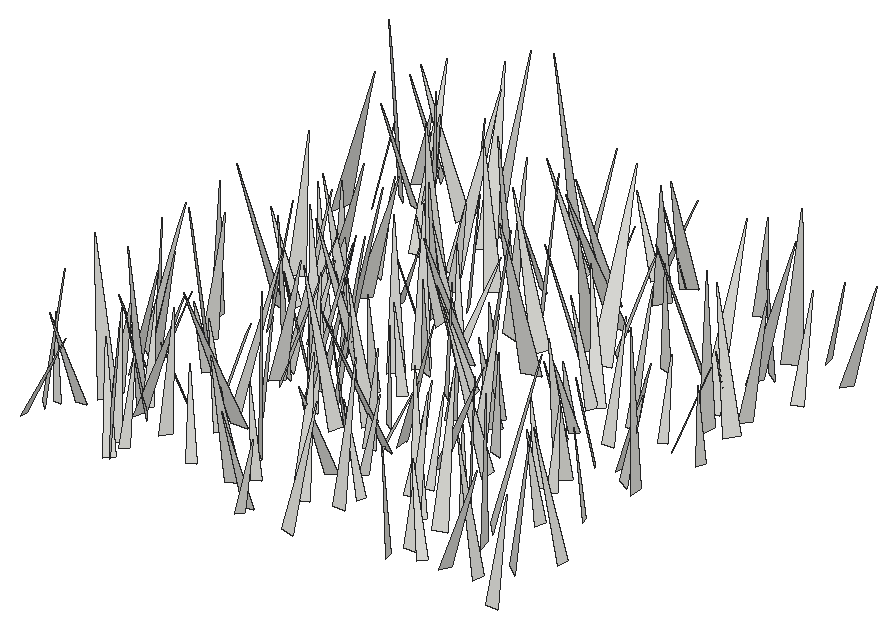
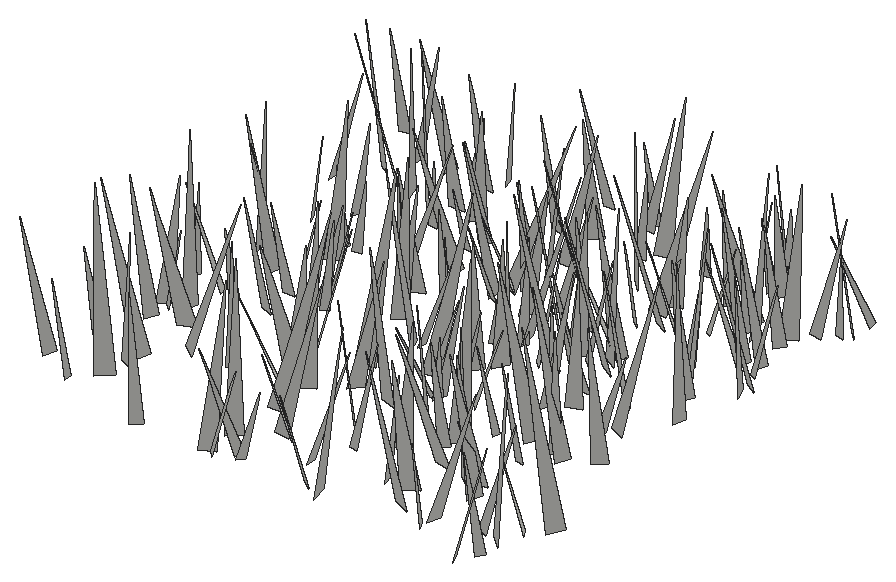
# SketchUp Ruby script. Lengths in inches.
U = 1.inch
M = Sketchup.active_model
def pt(a) = Geom::Point3d.new(a.map { |v| v * U })
def face(e, loops, mat)
  f = e.add_face(loops[0].map { |a| pt(a) })
  loops[1..].each { |l| e.add_face(l.map { |a| pt(a) }).erase! }
  f.material = f.back_material = mat if mat
  f
end
# faces: each face lists its corners as indices into pts; further lists are holes
def faces(e, pts, list, mat = nil) = list.each { |f| face(e, (f[0].is_a?(Array) ? f : [f]).map { |l| l.map { |i| pts[i] } }, mat) }
# xy, xz, yz: faces in a plane at the given z, y or x. An outline is a flat list of corners, or four numbers for a rectangle; further outlines are holes
def ring(l) = l.size == 4 ? [[l[0], l[1]], [l[2], l[1]], [l[2], l[3]], [l[0], l[3]]] : l.each_slice(2).to_a
def flat(e, list, mat, &to3) = list.each { |f| face(e, (f[0].is_a?(Array) ? f : [f]).map { |l| ring(l).map { |u, v| to3.(u, v) } }, mat) }
def xy(e, z, list, mat = nil) = flat(e, list, mat) { |x, y| [x, y, z] }
def xz(e, y, list, mat = nil) = flat(e, list, mat) { |x, z| [x, y, z] }
def yz(e, x, list, mat = nil) = flat(e, list, mat) { |y, z| [x, y, z] }
def lines(e, pts, list) = list.each { |a, b| e.add_line(pt(pts[a]), pt(pts[b])) }
# prism: a flat outline (further loops are holes) pulled along v
def prism(e, loops, v, mat = nil)
  f = face(e, loops, mat); d = Geom::Vector3d.new(v.map { |x| x * U })
  f.pushpull(f.normal.samedirection?(d) ? d.length : -d.length)
end
def box(e, o, s, mat = nil) = prism(e, [[o, [o[0] + s[0], o[1], o[2]], [o[0] + s[0], o[1] + s[1], o[2]], [o[0], o[1] + s[1], o[2]]]], [0, 0, s[2]], mat)
def at(x, y, z, deg = 0) = Geom::Transformation.translation(pt([x, y, z])) * Geom::Transformation.rotation(ORIGIN, Z_AXIS, deg.degrees)
def axes(o, x, y, z) = Geom::Transformation.new([*x, 0, *y, 0, *z, 0, *pt(o).to_a, 1])
def part(name) = M.definitions.add(name)
# library, detail: a bought-in or finely detailed component or shape, given as its bounding box
def library(name, o, s) = part(name).tap { |d| box(d.entities, o, s) }
def detail(e, o, s) = box(e.add_group.entities, o, s)
def put(e, d, t, mat = nil) = e.add_instance(d, t).tap { |i| i.material = mat if mat }
def group(e, t, mat = nil) = e.add_group.tap { |g| g.transformation = t; g.material = mat if mat }.entities
root = M.entities
c1 = part("fur_instance\#9")
p = [[0.8125,0,1.79],[0.67,-0.02,1.48],[0,-0.11,0],[0,0.11,0]]
faces(c1.entities,p,[[0,1,2,3]])
put(root,c1,axes([501.8,309.96,-21.66],[0.50374,3.60666,1.32904],[3.78488,-0.69911,0.46265],[-0.67011,-1.23747,3.61216]))
put(root,c1,axes([502.37,352.37,-21.66],[-4.94486,-5.49387,2.91837],[-6.02867,5.15162,-0.51692],[1.53451,2.53562,7.37341]))
put(root,c1,axes([501.12,309.07,-21.66],[4.60486,4.04407,1.88978],[4.30358,-4.74303,-0.33665],[-1.18533,-1.50984,6.1193]))
put(root,c1,axes([501.48,349.91,-21.66],[2.95559,2.2846,0.71516],[2.24296,-3.03986,0.44126],[-0.83663,-0.07885,3.70947]))
put(root,c1,axes([502.125,321.92,-21.66],[-4.83531,-1.63891,2.39644],[-2.01972,5.24312,-0.48946],[2.08559,1.27782,5.08199]))
put(root,c1,axes([503.12,356.64,-21.66],[-4.38014,-2.49103,0.91186],[-2.44951,4.47381,0.4553],[1.01814,0.04674,5.01832]))
put(root,c1,axes([499.65,348.23,-21.66],[8.0282,-2.33719,0.44231],[-2.30718,-8.02996,-0.55383],[-0.57877,-0.40914,8.34313]))
put(root,c1,axes([500.875,306.83,-21.66],[4.1398,0.29454,0.02134],[0.28882,-4.10074,0.57065],[-0.06159,0.56772,4.11084]))
put(root,c1,axes([503.16,319.11,-21.66],[-1.78915,-3.44674,0.35763],[-3.41457,1.82215,0.479],[0.59044,0.09337,3.85378]))
put(root,c1,axes([503.31,311.05,-21.66],[-0.2394,-4.99537,0.47277],[-5.01072,0.21306,-0.28607],[-0.26442,0.48521,4.99291]))
put(root,c1,axes([501.91,354.89,-21.66],[3.6262,-2.26105,0.60128],[-2.31235,-3.63241,0.28605],[-0.35624,0.56255,4.26378]))
put(root,c1,axes([501.99,320.76,-21.66],[3.861,5.57007,1.34937],[5.71182,-3.87341,-0.35436],[-0.47072,-1.31331,6.76812]))
put(root,c1,axes([504.14,351.86,-21.66],[-1.82389,-4.57282,0.8897],[-4.65371,1.74485,-0.5721],[-0.21262,1.03617,4.88978]))
put(root,c1,axes([503.1,328.43,-21.66],[6.40054,-0.55178,2.21578],[-0.37829,-6.75939,-0.5905],[-2.25189,-0.43282,6.39709]))
put(root,c1,axes([503.78,337.5625,-21.66],[3.27303,-4.65782,3.06275],[-5.40234,-3.52629,0.41046],[-1.37496,2.76738,5.67799]))
put(root,c1,axes([504.5625,312.82,-21.66],[-4.39266,5.33205,2.64396],[5.82364,4.52851,0.54275],[1.2274,-2.40386,6.88706]))
put(root,c1,axes([505.83,332.8,-21.66],[-2.53564,-6.45433,1.27855],[-6.57975,2.48748,-0.49186],[0.00081,1.3699,6.91708]))
put(root,c1,axes([503.45,317.55,-21.66],[5.71322,-0.96407,0.62556],[-0.92485,-5.73993,-0.39936],[-0.68221,-0.29224,5.7802]))
put(root,c1,axes([506.85,333.59,-21.66],[-3.73085,2.02538,0.45172],[2.07172,3.68874,0.57157],[0.11914,-0.71871,4.20651]))
put(root,c1,axes([504.38,314.13,-21.66],[3.71133,-3.4553,1.19556],[-3.62183,-3.7076,0.52772],[-0.50083,1.20708,5.04327]))
put(root,c1,axes([504.86,325.24,-21.66],[5.24676,-2.59436,1.90695],[-2.83441,-5.4512,0.38233],[-1.5275,1.20389,5.84064]))
put(root,c1,axes([505.79,323.85,-21.66],[-4.21383,-5.23135,2.06774],[-5.35043,4.52497,0.54449],[1.7365,1.24763,6.69529]))
put(root,c1,axes([508.29,352.72,-21.66],[-6.63907,0.80935,0.83748],[0.8673,6.67065,0.42894],[0.7773,-0.53025,6.67446]))
put(root,c1,axes([504.83,318.04,-21.66],[6.44965,-0.53992,1.19924],[-0.48241,-6.55498,-0.35669],[-1.22351,-0.26161,6.46237]))
put(root,c1,axes([506.85,314.2,-21.66],[-6.68895,-1.28776,2.75903],[-1.15,7.23488,0.5888],[2.81923,-0.10417,6.78629]))
put(root,c1,axes([504.95,318.47,-21.66],[4.62251,0.92588,0.22465],[0.9419,-4.60847,-0.38752],[-0.14333,-0.42437,4.69837]))
put(root,c1,axes([507.75,313.86,-21.66],[-3.18277,2.93848,0.48438],[2.88307,3.21784,-0.5768],[0.74643,0.10079,4.29324]))
put(root,c1,axes([507.36,338.56,-21.66],[1.49528,-4.80686,1.53266],[-5.04418,-1.45777,0.34917],[-0.10564,1.56838,5.02194]))
put(root,c1,axes([507.93,321.08,-21.66],[2.18541,-3.04998,0.78828],[-3.02604,-2.29919,-0.50659],[-0.87571,0.3334,3.71777]))
put(root,c1,axes([507.1875,329.8,-21.66],[5.44742,2.57642,1.57153],[2.74581,-5.57692,-0.37485],[-1.25227,-1.0208,6.0143]))
put(root,c1,axes([508.65,312.6,-21.66],[-3.91635,-3.27614,1.36892],[-3.24396,4.13005,0.60351],[1.44353,0.39293,5.07017]))
put(root,c1,axes([509.18,346.06,-21.66],[-1.39232,7.88876,0.40308],[7.89477,1.37627,0.33483],[-0.26016,-0.45487,8.00369]))
put(root,c1,axes([508.58,354.06,-21.66],[-3.28983,-1.54802,1.9149],[-2.00034,3.5437,-0.57187],[1.43591,1.38997,3.59058]))
put(root,c1,axes([509.24,307.79,-21.66],[3.60121,-2.60608,3.3834],[-3.59297,-4.24118,0.55747],[-2.30861,2.53545,4.41017]))
put(root,c1,axes([506.34,339,-21.66],[6.83641,-1.96558,0.32372],[-1.94381,-6.83529,-0.45298],[-0.43579,-0.34652,7.09893]))
put(root,c1,axes([508,347.98,-21.66],[5.45486,-2.53583,1.72286],[-2.73109,-5.61705,0.37948],[-1.39279,1.08278,6.00349]))
put(root,c1,axes([510.41,305.71,-21.66],[-3.8761,2.85036,0.12124],[2.83481,3.87102,-0.37744],[0.32105,0.23257,4.79648]))
put(root,c1,axes([509.23,345.9375,-21.66],[1.43263,3.39143,0.32506],[3.34277,-1.46736,0.57677],[-0.65831,-0.07043,3.63615]))
put(root,c1,axes([508.81,341.35,-21.66],[1.57919,4.13225,1.33364],[4.34025,-1.54395,-0.35548],[-0.12772,-1.37428,4.40942]))
put(root,c1,axes([510.11,316.02,-21.66],[-1.91573,-3.10975,0.18965],[-3.07242,1.92263,0.49017],[0.51647,-0.09744,3.61944]))
put(root,c1,axes([510.33,346.37,-21.66],[4.06784,5.47307,2.7985],[5.78633,-4.54195,0.47187],[-2.07475,-1.93641,6.80288]))
put(root,c1,axes([510.15,305.88,-21.66],[3.4021,4.35261,1.87369],[4.47593,-3.70904,0.48912],[-1.55627,-1.15238,5.50275]))
put(root,c1,axes([508.04,312.48,-21.66],[6.4862,-0.82849,0.61771],[-0.87391,-6.49276,0.46816],[-0.55158,0.54452,6.52212]))
put(root,c1,axes([510.38,307.6,-21.66],[-2.95191,2.4359,0.97471],[2.3622,3.10602,-0.60836],[1.1418,-0.12828,3.77853]))
put(root,c1,axes([510.95,331.84,-21.66],[-2.98056,5.41129,1.99239],[5.72855,3.03527,0.32601],[0.65987,-1.90801,6.16924]))
put(root,c1,axes([512.72,333.07,-21.66],[-6.49588,1.72746,1.45223],[1.82521,6.62397,0.28488],[1.32729,-0.65455,6.71561]))
put(root,c1,axes([510.625,334.0625,-21.66],[3.65523,2.01923,0.98653],[2.16689,-3.66612,-0.52479],[-0.59594,-0.94526,4.14277]))
put(root,c1,axes([511.65,311.2,-21.66],[4.3952,-2.19196,2.60814],[-2.70598,-4.83259,0.49862],[-2.06997,1.6632,4.88608]))
put(root,c1,axes([512.76,350.07,-21.66],[-3.64093,6.72533,0.73654],[6.73348,3.68347,-0.34805],[0.65778,-0.48058,7.63972]))
put(root,c1,axes([511.72,352.54,-21.66],[2.95959,7.19025,1.54721],[7.29869,-3.07695,0.338],[-0.90704,-1.29822,7.76818]))
put(root,c1,axes([511.7,329.4,-21.66],[0.71871,3.7725,0.80138],[3.83913,-0.62217,-0.51422],[0.36739,-0.87844,3.80576]))
put(root,c1,axes([510.1,337.96,-21.66],[6.42408,-3.63909,0.41323],[-3.66082,-6.40525,0.50369],[-0.11006,0.64215,7.36601]))
put(root,c1,axes([513.28,324.45,-21.66],[2.89079,5.81329,3.19782],[6.3896,-3.37876,0.3661],[-1.787,-2.67707,6.48205]))
put(root,c1,axes([512.63,325.57,-21.66],[3.66563,6.83822,1.35122],[6.90712,-3.76874,0.33492],[-0.93742,-1.02919,7.75151]))
put(root,c1,axes([512.125,317.5,-21.66],[3.35941,2.47012,0.56366],[2.52325,-3.34641,-0.37364],[-0.22894,-0.63632,4.15301]))
put(root,c1,axes([513.17,345.47,-21.66],[1.15921,7.66569,0.40932],[7.66684,-1.17697,0.3294],[-0.3873,-0.35503,7.74584]))
put(root,c1,axes([514.54,325.61,-21.66],[-2.99975,-3.60869,1.08185],[-3.74003,3.01886,-0.30041],[0.45307,1.02732,4.68304]))
put(root,c1,axes([514.78,314.26,-21.66],[2.55776,-3.86723,2.22173],[-4.13899,-3.01226,-0.47827],[-1.66143,1.55064,4.61182]))
put(root,c1,axes([513.9375,330.92,-21.66],[0.22689,-3.51122,0.97081],[-3.62685,-0.12635,0.39066],[0.3422,0.98893,3.49679]))
put(root,c1,axes([512.95,339.03,-21.66],[3.6641,-0.22277,0.06955],[-0.2117,-3.63329,-0.48425],[-0.09821,-0.47926,3.63879]))
put(root,c1,axes([514.47,341.83,-21.66],[-4.81324,5.46383,3.73935],[6.29264,5.21276,0.48307],[2.05886,-3.15867,7.26549]))
put(root,c1,axes([515.17,349.93,-21.66],[-5.00491,-0.78513,1.46412],[-0.94309,5.16869,-0.45214],[1.36772,0.69095,5.0459]))
put(root,c1,axes([513.02,323.53,-21.66],[5.25974,-3.61511,1.15521],[-3.73911,-5.27428,0.51907],[-0.65007,1.0869,6.36116]))
put(root,c1,axes([515.89,325.07,-21.66],[-4.29093,5.93832,1.73067],[6.14946,4.32229,0.41585],[0.66564,-1.65078,7.31456]))
put(root,c1,axes([515.29,315.96,-21.66],[-0.22294,-7.81188,0.28991],[-7.80547,0.20653,-0.4373],[-0.42917,0.30182,7.80282]))
put(root,c1,axes([513.73,317.39,-21.66],[3.6487,6.36792,1.23917],[6.47764,-3.65398,-0.29593],[-0.35515,-1.22351,7.3332]))
put(root,c1,axes([513.47,323.29,-21.66],[5.3948,4.35682,0.5893],[4.31887,-5.42625,0.57994],[-0.82254,0.08385,6.9101]))
put(root,c1,axes([516.04,308.92,-21.66],[-1.47936,3.73163,0.54523],[3.76451,1.42617,0.45319],[-0.22551,-0.67216,3.98851]))
put(root,c1,axes([515.53,318.36,-21.66],[2.40724,3.27999,1.19788],[3.2967,-2.61439,0.53362],[-1.15108,-0.62824,4.03341]))
put(root,c1,axes([514.95,343.09,-21.66],[2.82245,-3.27125,1.23973],[-3.47956,-2.78972,0.56063],[-0.36142,1.31172,4.28404]))
put(root,c1,axes([517.2,336.48,-21.66],[-2.83398,-2.56318,0.53676],[-2.6174,2.79801,-0.45803],[0.08496,0.70049,3.79362]))
put(root,c1,axes([516.24,339.42,-21.66],[5.75232,0.0292,2.58276],[0.25276,-6.28131,-0.49192],[-2.57052,-0.55229,5.73133]))
put(root,c1,axes([515.87,325.9,-21.66],[3.90442,0.1948,1.09665],[0.0575,-4.02752,0.51071],[-1.11233,0.47558,3.87577]))
put(root,c1,axes([517.37,345.14,-21.66],[-3.57367,4.96866,1.72232],[5.21894,3.60663,0.42422],[0.64547,-1.65218,6.10563]))
put(root,c1,axes([517.49,338.39,-21.66],[-4.79801,0.15244,1.14259],[0.25589,4.91001,0.4195],[1.12396,-0.46714,4.78206]))
put(root,c1,axes([517.96,355.15,-21.66],[-7.87878,-1.52664,2.20407],[-1.70967,8.13085,-0.47967],[2.06533,0.90687,8.01097]))
put(root,c1,axes([515.21,328.88,-21.66],[7.84011,2.17766,1.89393],[2.14429,-8.06482,0.39652],[-1.93163,-0.114,8.12726]))
put(root,c1,axes([517.49,328.16,-21.66],[-3.40896,-3.60182,1.17644],[-3.63778,3.55381,0.3393],[1.06005,0.61272,4.94762]))
put(root,c1,axes([516.375,324.13,-21.66],[1.54796,-4.76639,0.70367],[-4.81569,-1.50748,0.38266],[0.1508,0.78667,4.99682]))
put(root,c1,axes([518.24,321.28,-21.66],[-0.17119,5.69768,1.30234],[5.83131,0.07859,0.42267],[-0.39436,-1.31119,5.68456]))
put(root,c1,axes([517.51,341.92,-21.66],[4.70905,2.28139,1.77217],[2.5251,-4.89691,-0.40574],[-1.40329,-1.15586,5.21682]))
put(root,c1,axes([520.57,325.68,-21.66],[-7.92829,-1.68885,1.19775],[-1.65667,8.01779,0.33921],[1.24187,-0.08605,8.09907]))
put(root,c1,axes([519.56,330.26,-21.66],[-5.3119,3.70536,1.5571],[3.75007,5.49761,-0.28937],[1.44609,-0.64586,6.4701]))
put(root,c1,axes([517.63,321.12,-21.66],[5.42391,5.6075,1.42758],[5.74422,-5.4537,-0.40246],[-0.69711,-1.3092,7.79108]))
put(root,c1,axes([519.43,313.35,-21.66],[4.46233,4.90899,2.88894],[5.22756,-4.98695,0.39938],[-2.26203,-1.84084,6.62202]))
put(root,c1,axes([520.18,337.37,-21.66],[-3.13044,2.30171,0.23571],[2.28042,3.13636,-0.34054],[0.39127,0.13578,3.8706]))
put(root,c1,axes([520.18,337.02,-21.66],[-5.09295,0.86723,1.4086],[1.03106,5.23004,0.50795],[1.29351,-0.75432,5.14123]))
put(root,c1,axes([521.53,320.25,-21.66],[-6.69944,1.03913,0.45559],[1.00559,6.70154,-0.49804],[0.5255,0.42362,6.76123]))
put(root,c1,axes([518.79,323.71,-21.66],[4.76999,5.26227,1.90717],[5.37132,-5.00824,0.38463],[-1.57405,-1.14351,7.09199]))
put(root,c1,axes([520.79,331.95,-21.66],[-5.28353,4.19242,1.51467],[4.2139,5.46353,-0.42331],[1.45386,-0.59977,6.73148]))
put(root,c1,axes([519.55,354.6,-21.66],[2.50571,3.8301,0.73521],[3.84486,-2.57244,0.29737],[-0.65369,-0.44905,4.56726]))
put(root,c1,axes([521.66,351.48,-21.66],[-5.37487,-0.5228,0.79074],[-0.44432,5.41107,0.55741],[0.83736,-0.48456,5.37139]))
put(root,c1,axes([520.36,347.75,-21.66],[-1.29347,-4.18784,0.40951],[-4.17089,1.33267,0.45438],[0.55623,0.25449,4.35943]))
put(root,c1,axes([520.32,326.58,-21.66],[3.95695,-1.9726,1.7752],[-1.97238,-4.31833,-0.40205],[-1.77544,0.40099,4.40306]))
put(root,c1,axes([520.65,308.54,-21.66],[2.01145,-6.31603,1.30369],[-6.40118,-2.12156,-0.40211],[-0.78536,1.11557,6.61638]))
put(root,c1,axes([521.75,309.97,-21.66],[-1.38179,3.78074,1.32931],[4.00762,1.30133,0.46468],[-0.00636,-1.40818,3.99842]))
put(root,c1,axes([520.61,337.45,-21.66],[0.96645,3.75371,0.08435],[3.72936,-0.9496,-0.47076],[0.43512,-0.19848,3.84744]))
put(root,c1,axes([522.22,327.74,-21.66],[-1.64307,3.38565,0.94063],[3.51296,1.55882,0.52563],[-0.08077,-1.0745,3.72639]))
put(root,c1,axes([521.48,331.61,-21.66],[-0.96334,-4.21277,1.52504],[-4.43315,1.12201,0.29911],[0.64835,1.41239,4.31115]))
put(root,c1,axes([522.96,334.24,-21.66],[-3.66432,1.46778,0.50332],[1.5223,3.65057,0.437],[0.30055,-0.59495,3.9231]))
put(root,c1,axes([523.24,322.42,-21.66],[-5.24229,2.67543,1.59997],[2.88849,5.34612,0.52444],[1.17239,-1.20849,5.86212]))
put(root,c1,axes([522.4375,344.97,-21.66],[-3.91577,-3.49387,3.17429],[-4.26524,4.38586,-0.43413],[2.02262,2.48468,5.2299]))
put(root,c1,axes([522.86,340.33,-21.66],[2.04699,7.14679,2.15899],[7.40344,-2.23185,0.36858],[-0.96272,-1.9673,7.42502]))
put(root,c1,axes([522.91,334.78,-21.66],[1.39715,-7.46285,0.32526],[-7.45597,-1.41344,-0.40331],[-0.45656,0.24497,7.58179]))
put(root,c1,axes([524.07,306.0625,-21.66],[-0.19346,-4.85951,0.89963],[-4.92735,0.1202,-0.41034],[-0.38132,0.91231,4.84602]))
put(root,c1,axes([524.45,323.28,-21.66],[2.05844,3.54151,1.67651],[3.74882,-2.33096,0.32115],[-1.13989,-1.27062,4.08367]))
put(root,c1,axes([526.38,339.98,-21.66],[-5.76808,3.66085,1.08427],[3.77252,5.76709,0.59739],[0.58783,-1.08949,6.80556]))
put(root,c1,axes([524.06,304.99,-21.66],[3.08181,-1.73974,0.98019],[-1.88437,-3.1302,0.36886],[-0.66077,0.81254,3.51969]))
put(root,c1,axes([525.01,329.79,-21.66],[2.79154,3.79561,1.789],[3.98615,-3.06992,0.29332],[-1.31064,-1.25251,4.70248]))
put(root,c1,axes([526.23,354.59,-21.66],[-3.21224,1.96871,0.46482],[2.01704,3.18335,0.45637],[0.15311,-0.63315,3.7398]))
put(root,c1,axes([525.2,317.47,-21.66],[-3.25628,-4.53556,1.56998],[-4.60157,3.48952,0.53691],[1.36443,0.94415,5.55755]))
put(root,c1,axes([526.51,331.47,-21.66],[-4.93591,-0.64757,0.62999],[-0.58328,4.95621,0.52453],[0.68994,-0.44273,4.95049]))
put(root,c1,axes([526.71,320.17,-21.66],[-3.06964,-6.81398,0.3454],[-6.81954,3.05272,-0.38339],[-0.20825,0.47214,7.46364]))
put(root,c1,axes([526.15,349.53,-21.66],[-0.27695,-6.43694,1.01641],[-6.49492,0.18954,-0.56932],[-0.53231,1.03627,6.4177]))
put(root,c1,axes([525.81,314.4375,-21.66],[1.38462,-5.25865,0.1546],[-5.22749,-1.39323,-0.57157],[-0.5921,0.00308,5.40776]))
put(root,c1,axes([525.53,319.41,-21.66],[2.1664,-3.98299,1.68795],[-4.30586,-2.16689,0.41322],[-0.41582,1.68731,4.51516]))
put(root,c1,axes([526.5625,309.56,-21.66],[-2.92394,5.35838,1.35906],[5.44647,3.05552,-0.32925],[0.94614,-1.02969,6.09534]))
put(root,c1,axes([525.11,349.6,-21.66],[2.99336,2.37967,0.42143],[2.41657,-2.95437,-0.48225],[-0.02533,-0.63994,3.79348]))
put(root,c1,axes([526.73,322.29,-21.66],[1.45638,3.8911,0.37542],[3.87774,-1.48869,0.38679],[-0.49475,-0.21394,4.13668]))
put(root,c1,axes([528.625,355.3,-21.66],[-2.84095,-2.72325,0.75235],[-2.80656,2.8428,-0.30791],[0.32453,0.74533,3.9233]))
put(root,c1,axes([526.33,320.05,-21.66],[3.11612,2.14822,0.04863],[2.13222,-3.08072,-0.53874],[0.26618,-0.47091,3.74631]))
put(root,c1,axes([526.97,331.92,-21.66],[6.97385,3.06548,2.09729],[3.25235,-7.19468,-0.2986],[-1.79388,-1.12684,7.61201]))
put(root,c1,axes([528.1,336.64,-21.66],[1.76512,-7.95634,1.31885],[-8.03843,-1.84494,-0.37166],[-0.65291,1.20466,8.14131]))
put(root,c1,axes([527.83,315.89,-21.66],[3.18405,-1.52738,1.26596],[-1.78098,-3.25535,0.55182],[-0.87386,1.06936,3.48806]))
put(root,c1,axes([526.91,353.97,-21.66],[4.6922,-0.3007,0.23761],[-0.32477,-4.66947,0.50417],[-0.20347,0.51889,4.67471]))
put(root,c1,axes([530.08,312.79,-21.66],[-3.96056,0.86775,0.15545],[0.85071,3.94968,-0.37345],[0.23119,0.33194,4.03727]))
put(root,c1,axes([528.875,346.65,-21.66],[0.62863,-8.27068,0.12443],[-8.26435,-0.63324,-0.33804],[-0.34653,0.09834,8.28764]))
put(root,c1,axes([527.08,321.69,-21.66],[6.44978,-0.00096,0.92482],[0.04605,-6.50733,-0.32793],[-0.92367,-0.33115,6.44144]))
put(root,c1,axes([527.71,326.99,-21.66],[2.72527,-3.47225,0.02549],[-3.46346,-2.7159,0.33551],[0.24824,0.22715,4.40125]))
put(root,c1,axes([529.59,310.55,-21.66],[0.8824,6.11345,1.2337],[6.18895,-1.01221,0.58924],[-0.77016,-1.12963,6.14863]))
put(root,c1,axes([528.84,305.04,-21.66],[0.94432,5.62245,1.27282],[5.76049,-0.87093,-0.42662],[0.22085,-1.32412,5.68522]))
put(root,c1,axes([531.12,339.625,-21.66],[-4.99483,-3.69291,1.05885],[-3.66459,5.10128,0.50484],[1.15306,0.21561,6.19121]))
put(root,c1,axes([529.18,355.1,-21.66],[3.47226,-5.91321,0.27335],[-5.89868,-3.48291,-0.41506],[-0.49636,0.02495,6.84473]))
put(root,c1,axes([529.03,351.89,-21.66],[5.34448,-4.72432,0.68412],[-4.69665,-5.3877,-0.51471],[-0.85369,0.0645,7.11462]))
put(root,c1,axes([531.41,341.23,-21.66],[-2.88963,7.72101,0.14725],[7.7077,2.8933,-0.45358],[0.4764,0.02131,8.23153]))
put(root,c1,axes([529.3,342.47,-21.66],[4.72004,-5.82808,0.22381],[-5.80637,-4.72269,-0.52693],[-0.55017,-0.15829,7.48115]))
put(root,c1,axes([530.48,329.23,-21.66],[4.51111,-4.76568,1.07484],[-4.75985,-4.61702,-0.49408],[-1.1004,0.43419,6.54353]))
put(root,c1,axes([531.24,328.16,-21.66],[2.7716,-4.32676,0.73791],[-4.29866,-2.85215,-0.57784],[-0.88707,0.30254,5.10575]))
put(root,c1,axes([531.25,343.32,-21.66],[3.44436,3.22324,0.28553],[3.18394,-3.45028,0.54084],[-0.57733,0.20181,4.68619]))
put(root,c1,axes([531.97,325.06,-21.66],[-1.06035,5.5551,1.84187],[5.77115,1.30347,-0.60889],[0.97234,-1.67863,5.62252]))
put(root,c1,axes([533.375,317.26,-21.66],[-0.09668,3.9627,0.07364],[3.92699,0.08582,0.53775],[-0.5359,-0.08606,3.92724]))
put(root,c1,axes([535.43,321.99,-21.66],[-7.05219,-0.0174,0.36445],[-0.04272,7.04446,-0.49029],[0.36236,0.49184,7.03515]))
put(root,c1,axes([532.85,315.54,-21.66],[-1.4542,4.67664,1.33998],[4.76533,1.65076,-0.58976],[0.97884,-1.08869,4.86188]))
put(root,c1,axes([535.46,335.71,-21.66],[-3.60755,4.52257,0.00535],[4.517,3.60276,0.29145],[-0.22451,-0.18592,5.77782]))
put(root,c1,axes([535.18,335.32,-21.66],[-4.286,2.05614,0.85108],[2.13965,4.31523,0.34994],[0.6115,-0.68765,4.74078]))
put(root,c1,axes([533.83,324.9,-21.66],[0.99186,4.25892,2.03749],[4.71935,-0.95274,-0.30591],[-0.13232,-2.05608,4.36218]))
put(root,c1,axes([531.8,320.4375,-21.66],[5.92157,-1.3609,0.111],[-1.36516,-5.91048,0.36315],[-0.02664,0.3788,6.06507]))
put(root,c1,axes([535.6,312.99,-21.66],[-5.07407,3.61415,0.85454],[3.5922,5.14344,-0.42375],[0.94256,-0.14624,6.2152]))
put(root,c1,axes([536.02,331.76,-21.66],[2.32734,-2.83374,0.7234],[-2.82694,-2.41664,-0.37171],[-0.74954,0.31569,3.64807]))
put(root,c1,axes([536.98,329.82,-21.66],[-3.57828,-1.18752,0.86435],[-1.11493,3.67791,0.43741],[0.95617,-0.15551,3.74473]))
put(root,c1,axes([535.97,343.69,-21.66],[-0.76363,-5.08076,1.72351],[-5.30047,0.98391,0.55201],[0.83046,1.60796,5.10809]))
put(root,c1,axes([536.47,331.52,-21.66],[1.6071,-3.85332,0.26864],[-3.82652,-1.62792,-0.45895],[-0.52725,0.06941,4.14972]))
put(root,c1,axes([537.44,306.97,-21.66],[-4.30965,-1.39305,1.63599],[-1.58025,4.5392,-0.29767],[1.45598,0.80324,4.51941]))
put(root,c1,axes([537.79,316.02,-21.66],[-0.46969,3.55211,0.73396],[3.59032,0.35011,0.60316],[-0.51554,-0.79795,3.53189]))
put(root,c1,axes([538.04,312.64,-21.66],[-1.0825,6.58238,0.66021],[6.6005,1.02978,0.55528],[-0.44383,-0.73975,6.64764]))
put(root,c1,axes([536.24,355.22,-21.66],[2.86346,-4.49186,1.0378],[-4.60706,-2.8331,0.44926],[-0.16992,1.11803,5.30796]))
put(root,c1,axes([538.19,308.8,-21.66],[-0.0106,6.43156,0.96228],[6.47441,-0.07994,0.60561],[-0.61077,-0.95901,6.403]))
put(root,c1,axes([539.91,308.12,-21.66],[-2.40389,3.30252,0.08348],[3.28439,2.37806,0.4999],[-0.35549,-0.36124,4.05406]))
put(root,c1,axes([540.28,343.59,-21.66],[-3.80657,-5.75041,0.9295],[-5.82495,3.76407,-0.56819],[0.03325,1.08891,6.87272]))
put(root,c1,axes([539.85,323,-21.66],[-1.79664,3.17113,0.9039],[3.29721,1.71578,0.53432],[-0.03822,-1.04932,3.60534]))
put(root,c1,axes([539.83,331.5625,-21.66],[0.07202,5.27236,0.64208],[5.29211,-0.12578,0.43929],[-0.45123,-0.63374,5.25452]))
put(root,c1,axes([539.5625,334.71,-21.66],[1.82838,5.64567,1.15342],[5.69001,-1.95997,0.57384],[-0.90985,-0.91206,5.90655]))
put(root,c1,axes([539.35,314.73,-21.66],[5.6621,3.46946,2.68851],[3.90579,-5.98471,-0.5026],[-2.00251,-1.86297,6.62147]))
put(root,c1,axes([541,328.4,-21.66],[-2.98198,-2.20876,0.85448],[-2.34628,2.94214,-0.58291],[0.32208,0.98295,3.66484]))
put(root,c1,axes([540.54,325.11,-21.66],[3.54462,-5.56954,2.15269],[-5.7416,-3.86654,-0.54956],[-1.63946,1.49942,6.57891]))
put(root,c1,axes([541.16,322.91,-21.66],[-2.54986,2.80817,1.27437],[2.87177,2.76487,-0.34653],[1.12374,-0.69377,3.77724]))
put(root,c1,axes([542.3,312.96,-21.66],[5.88559,1.89129,2.87248],[1.95642,-6.52369,0.2867],[-2.82853,-0.57687,6.17535]))
put(root,c1,axes([542.8125,340.58,-21.66],[-2.31741,7.72302,0.72504],[7.71845,2.37113,-0.58682],[0.77216,-0.52327,8.04183]))
put(root,c1,axes([541.03,315.46,-21.66],[5.81873,5.70667,1.51485],[5.84557,-5.86726,-0.35074],[-0.83073,-1.31442,8.14252]))
put(root,c1,axes([542.9375,334.57,-21.66],[-2.61192,2.51011,0.78878],[2.46687,2.72278,-0.49597],[0.91509,-0.17543,3.58843]))
put(root,c1,axes([543.62,318.31,-21.66],[-3.82053,1.38738,1.41647],[1.59253,3.97908,0.39802],[1.18113,-0.87734,4.0451]))
put(root,c1,axes([543.04,348.17,-21.66],[-2.5079,-4.6968,1.95628],[-4.90602,2.8103,0.45782],[1.34828,1.48955,5.3047]))
put(root,c1,axes([545.16,308.63,-21.66],[-5.94659,0.26274,1.16381],[0.1992,6.05181,-0.34844],[1.17635,0.30341,5.94219]))
put(root,c1,axes([542.13,308.21,-21.66],[5.3173,-1.56529,0.48292],[-1.59322,-5.32309,0.28875],[-0.38078,0.41424,5.53538]))
put(root,c1,axes([542.99,350.7,-21.66],[4.39252,-6.51911,2.0007],[-6.79057,-4.39945,0.57342],[-0.62428,1.98542,7.83991]))
put(root,c1,axes([542.5,346.69,-21.66],[7.35605,-1.97253,1.00478],[-2.03855,-7.39535,0.40615],[-0.86301,0.65556,7.60509]))
put(root,c1,axes([544.48,338.14,-21.66],[7.21029,-1.27081,2.71678],[-1.16788,-7.70491,-0.50453],[-2.76259,-0.05954,7.30402]))
put(root,c1,axes([543.05,329.4375,-21.66],[6.29896,-1.22347,0.37639],[-1.1888,-6.29213,-0.55798],[-0.47466,-0.47719,6.39237]))
put(root,c1,axes([545.92,320.98,-21.66],[-3.70453,-1.18645,1.17686],[-1.32576,3.8289,-0.31316],[1.01735,0.66938,3.87726]))
put(root,c1,axes([545.98,339.09,-21.66],[-2.17091,-2.72609,1.07786],[-2.90812,2.17161,-0.36485],[0.36901,1.07644,3.46573]))
put(root,c1,axes([546.6,338.7,-21.66],[-4.49758,4.50366,1.60112],[4.72062,4.53017,0.51777],[0.74986,-1.50644,6.34374]))
put(root,c1,axes([544.67,327.41,-21.66],[2.00613,4.44684,1.43472],[4.67253,-1.91449,-0.59961],[-0.01581,-1.5549,4.84142]))
put(root,c1,axes([546.21,327.125,-21.66],[-6.67663,-0.80436,2.4344],[-1.05353,7.05179,-0.55944],[2.33738,0.88086,6.7016]))
put(root,c1,axes([545,352.87,-21.66],[4.1341,0.32333,0.78637],[0.3951,-4.18703,-0.35553],[-0.75288,-0.42186,4.13146]))
put(root,c1,axes([544.1875,334.43,-21.66],[4.46845,1.48023,0.19389],[1.49287,-4.43008,-0.58427],[0.00126,-0.6156,4.67084]))
put(root,c1,axes([546,341.12,-21.66],[5.31281,-2.73186,1.51927],[-2.91837,-5.40827,0.48055],[-1.11999,1.13346,5.95467]))
put(root,c1,axes([548.85,314.64,-21.66],[-5.68888,-0.08485,0.69236],[-0.12916,5.71868,-0.36046],[0.68548,0.37338,5.67808]))
put(root,c1,axes([547.43,345.87,-21.66],[-2.09366,4.25191,0.8072],[4.26644,2.17826,-0.40798],[0.72654,-0.53866,4.72184]))
put(root,c1,axes([546.47,311.27,-21.66],[-3.30417,-4.76212,3.2823],[-5.25525,4.05058,0.5865],[2.41528,2.29867,5.7664]))
put(root,c1,axes([547.47,333.67,-21.66],[3.35457,-1.66316,1.27005],[-1.64462,-3.57909,-0.343],[-1.29397,0.23728,3.72849]))
put(root,c1,axes([548.88,305.63,-21.66],[-0.27729,4.76979,1.49646],[4.98187,0.38774,-0.31274],[0.41383,-1.47171,4.7676]))
put(root,c1,axes([548.5625,350.65,-21.66],[5.12871,-2.48578,0.55768],[-2.53054,-5.11559,0.47007],[-0.29413,0.66743,5.67995]))
